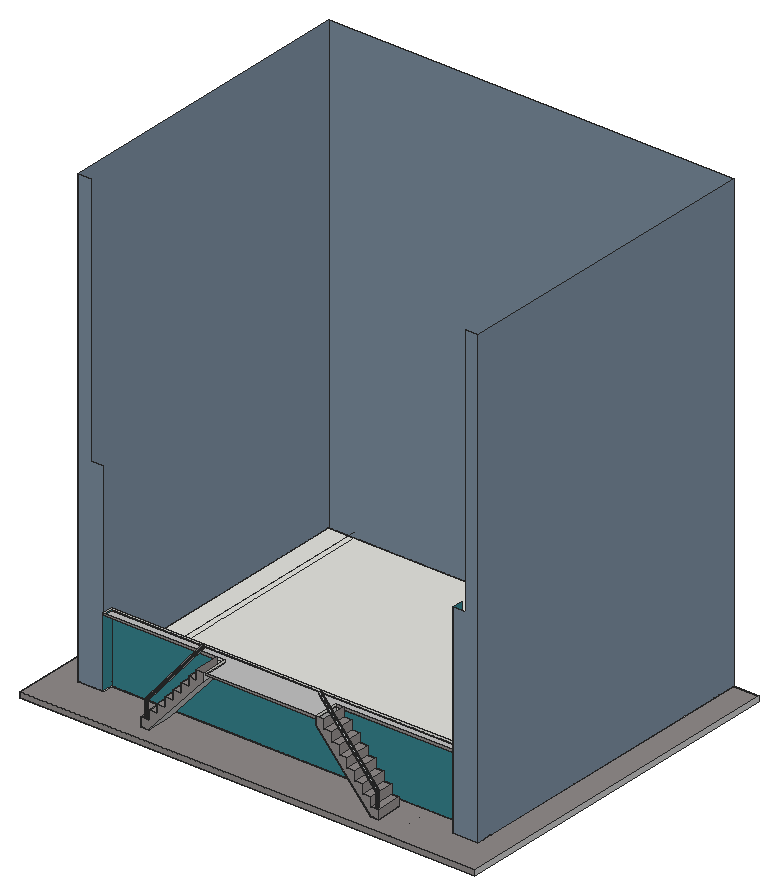
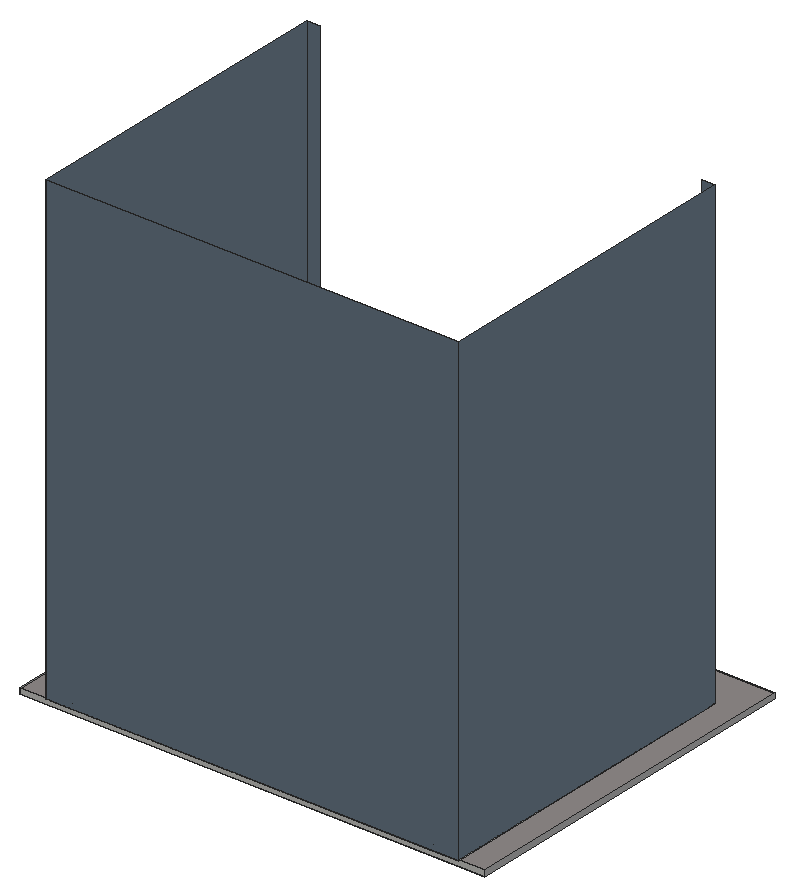
# SketchUp Ruby script. Lengths in inches.
U = 1.inch
M = Sketchup.active_model
def pt(a) = Geom::Point3d.new(a.map { |v| v * U })
def face(e, loops, mat)
  f = e.add_face(loops[0].map { |a| pt(a) })
  loops[1..].each { |l| e.add_face(l.map { |a| pt(a) }).erase! }
  f.material = f.back_material = mat if mat
  f
end
# faces: each face lists its corners as indices into pts; further lists are holes
def faces(e, pts, list, mat = nil) = list.each { |f| face(e, (f[0].is_a?(Array) ? f : [f]).map { |l| l.map { |i| pts[i] } }, mat) }
# xy, xz, yz: faces in a plane at the given z, y or x. An outline is a flat list of corners, or four numbers for a rectangle; further outlines are holes
def ring(l) = l.size == 4 ? [[l[0], l[1]], [l[2], l[1]], [l[2], l[3]], [l[0], l[3]]] : l.each_slice(2).to_a
def flat(e, list, mat, &to3) = list.each { |f| face(e, (f[0].is_a?(Array) ? f : [f]).map { |l| ring(l).map { |u, v| to3.(u, v) } }, mat) }
def xy(e, z, list, mat = nil) = flat(e, list, mat) { |x, y| [x, y, z] }
def xz(e, y, list, mat = nil) = flat(e, list, mat) { |x, z| [x, y, z] }
def yz(e, x, list, mat = nil) = flat(e, list, mat) { |y, z| [x, y, z] }
def lines(e, pts, list) = list.each { |a, b| e.add_line(pt(pts[a]), pt(pts[b])) }
# prism: a flat outline (further loops are holes) pulled along v
def prism(e, loops, v, mat = nil)
  f = face(e, loops, mat); d = Geom::Vector3d.new(v.map { |x| x * U })
  f.pushpull(f.normal.samedirection?(d) ? d.length : -d.length)
end
def box(e, o, s, mat = nil) = prism(e, [[o, [o[0] + s[0], o[1], o[2]], [o[0] + s[0], o[1] + s[1], o[2]], [o[0], o[1] + s[1], o[2]]]], [0, 0, s[2]], mat)
def at(x, y, z, deg = 0) = Geom::Transformation.translation(pt([x, y, z])) * Geom::Transformation.rotation(ORIGIN, Z_AXIS, deg.degrees)
def axes(o, x, y, z) = Geom::Transformation.new([*x, 0, *y, 0, *z, 0, *pt(o).to_a, 1])
def part(name) = M.definitions.add(name)
# library, detail: a bought-in or finely detailed component or shape, given as its bounding box
def library(name, o, s) = part(name).tap { |d| box(d.entities, o, s) }
def detail(e, o, s) = box(e.add_group.entities, o, s)
def put(e, d, t, mat = nil) = e.add_instance(d, t).tap { |i| i.material = mat if mat }
def group(e, t, mat = nil) = e.add_group.tap { |g| g.transformation = t; g.material = mat if mat }.entities
root = M.entities
M.materials.add("[0083_DarkTurquoise]").color = [52, 127, 137]
M.materials.add("[0110_LightSlateGray]").color = [119, 136, 153]
M.materials.add("[0131_Silver]").color = [192, 192, 192]
M.materials.add("[Steel Brushed Stainless]").color = [183, 187, 190]
M.materials.add("[Stone Marble]").color = [143, 138, 136]
xy(root,-12,[[0,0,1080,841.201]])
xy(root,0,[[60,97.201,120,121.201],[960,97.201,1020,121.201],[60,121.201,120,841.201],[120,121.201,960,841.201],[960,121.201,1020,841.201]])
xy(root,0.499,[[960,83.889,1020,97.201]])
xy(root,0.499,[[[0,0,1080,0,1080,841.201,1020,841.201,1020,83.889,960,83.889,960,121.201,120,121.201,120,97.201,60,97.201,60,841.201,0,841.201],[258.4,36.241,277.1,97.201],[802.9,37.201,821.6,98.161]]],"[Stone Marble]")
xy(root,0.5,[[258.4,36.241,277.1,97.201],[802.9,37.201,821.6,98.161]])
xy(root,21.4375,[[266.14,39.152,265.375,39.322,264.68,39.683,264.103,40.213,263.682,40.873,263.447,41.62,263.413,42.403,263.583,43.167,263.945,43.862,264.474,44.439,265.134,44.86,265.881,45.095,266.664,45.129,267.428,44.959,268.123,44.598,268.7,44.068,269.121,43.408,269.356,42.661,269.39,41.878,269.221,41.114,268.859,40.419,268.329,39.842,267.669,39.421,266.922,39.186]])
xy(root,21.4375,[[[258.4,36.241,277.1,97.201],[266.14,39.152,265.375,39.322,264.68,39.683,264.103,40.213,263.682,40.873,263.447,41.62,263.413,42.403,263.583,43.167,263.945,43.862,264.474,44.439,265.134,44.86,265.881,45.095,266.664,45.129,267.428,44.959,268.123,44.598,268.7,44.068,269.121,43.408,269.356,42.661,269.39,41.878,269.221,41.114,268.859,40.419,268.329,39.842,267.669,39.421,266.922,39.186]],[[802.9,37.201,821.6,98.161],[814.759,38.369,813.977,38.406,813.231,38.643,812.571,39.066,812.044,39.645,811.684,40.34,811.516,41.105,811.553,41.887,811.79,42.634,812.213,43.293,812.792,43.821,813.487,44.181,814.252,44.348,815.034,44.312,815.781,44.074,816.44,43.652,816.968,43.073,817.328,42.377,817.495,41.612,817.459,40.83,817.221,40.084,816.799,39.424,816.22,38.897,815.524,38.537]]],"[Stone Marble]")
xy(root,42.375,[[277.1,36.241,295.8,97.201],[784.2,37.201,802.9,98.161]],"[Stone Marble]")
xy(root,63.3125,[[295.8,36.241,314.5,97.201],[765.5,37.201,784.2,98.161]],"[Stone Marble]")
xy(root,84.25,[[314.5,36.241,333.2,97.201],[746.8,37.201,765.5,98.161]],"[Stone Marble]")
xy(root,105.1875,[[333.2,36.241,351.9,97.201],[728.1,37.201,746.8,98.161]],"[Stone Marble]")
xy(root,126.125,[[351.9,36.241,370.6,97.201],[709.4,37.201,728.1,98.161]],"[Stone Marble]")
xy(root,147.0625,[[370.6,36.241,389.3,97.201],[690.7,37.201,709.4,98.161]],"[Stone Marble]")
xy(root,162,[[408,37.201,408,97.201,120,97.201,120,121.201,960,121.201,960,97.201,672,97.201,672,37.201]],"[0131_Silver]")
xz(root,0,[[900,0.497,902.927,0.499,876,0.499],[875.998,0.499,875.998,0.5,876,0.499],[875.998,0.499,876,0.499,875.998,0.5],[876,0.499,875.998,0.5,876,0.5],[876,0.499,876,0.5,875.998,0.5],
  [876,0.499,876,0.5,875.998,0.5]])
xz(root,0,[[0,-12,1080,-12,1080,0.499,902.927,0.499,900,0.497,876,0.499,0,0.499]],"[Stone Marble]")
xz(root,36.241,[[258.4,0.499,277.1,0.5]])
xz(root,36.241,[[258.4,0.5,277.1,0.5,408,149.389,408,168,389.3,168,389.3,147.0625,370.6,147.0625,370.6,126.125,351.9,126.125,351.9,105.1875,333.2,105.1875,333.2,84.25,314.5,84.25,314.5,63.3125,295.8,63.3125,295.8,42.375,277.1,42.375,277.1,21.4375,258.4,21.4375]],"[Stone Marble]")
xz(root,37.201,[[802.9,0.499,821.6,0.5]])
xz(root,37.201,[[802.9,0.5,821.6,0.5,821.6,21.4375,802.9,21.4375,802.9,42.375,784.2,42.375,784.2,63.3125,765.5,63.3125,765.5,84.25,746.8,84.25,746.8,105.1875,728.1,105.1875,728.1,126.125,709.4,126.125,709.4,147.0625,690.7,147.0625,690.7,168,672,168,672,149.389],[408,162,672,168]],"[Stone Marble]")
xz(root,83.889,[[960,0.499,1020,0.499,1020,1080,990,1080,990,480,960,480]],"[0110_LightSlateGray]")
xz(root,97.201,[[60,0,120,0.499],[960,0,1020,0.499],[258.4,0.499,277.1,0.5],[258.4,0.5,258.4,21.4375,277.1,21.4375,277.1,42.375,295.8,42.375,295.8,63.3125,314.5,63.3125,314.5,84.25,333.2,84.25,333.2,105.1875,351.9,105.1875,351.9,126.125,370.6,126.125,370.6,147.0625,389.3,147.0625,389.3,162,408,162,408,149.389,277.1,0.5],[389.3,162,408,168]])
xz(root,97.201,[[60,0.499,120,0.499,120,480,90,480,90,1080,60,1080]],"[0110_LightSlateGray]")
xz(root,97.201,[[120,162,389.3,168],[672,162,960,168]],"[Stone Marble]")
xz(root,98.161,[[802.9,0.499,821.6,0.5],[802.9,0.5,672,149.389,672,162,690.7,162,690.7,147.0625,709.4,147.0625,709.4,126.125,728.1,126.125,728.1,105.1875,746.8,105.1875,746.8,84.25,765.5,84.25,765.5,63.3125,784.2,63.3125,784.2,42.375,802.9,42.375,802.9,21.4375,821.6,21.4375,821.6,0.5],[672,162,690.7,168]])
xz(root,121.201,[[120,0,960,0.499],[120,162,960,162,960,168,672,168,672,167.95,648,167.95,648,168,120,168]])
xz(root,121.201,[[120,0.499,960,162]],"[0083_DarkTurquoise]")
xz(root,841.201,[[0,-12,0,0.499,60,0.499,60,0,1020,0,1020,0.499,1080,0.499,1080,-12]])
xz(root,841.201,[[60,0,1020,1080]],"[0110_LightSlateGray]")
yz(root,0,[[0,-12,841.201,0.499]],"[0131_Silver]")
yz(root,60,[[97.201,0,121.201,0.499],[121.201,0,841.201,0.499]])
yz(root,60,[[97.201,0.499,841.201,1080]],"[0110_LightSlateGray]")
yz(root,120,[[97.201,0,121.201,0.499],[97.201,162,121.201,168]])
yz(root,120,[[97.201,0.499,121.201,162]],"[0083_DarkTurquoise]")
yz(root,258.4,[[36.241,0.499,97.201,0.5]])
yz(root,258.4,[[36.241,0.5,97.201,21.4375]],"[Stone Marble]")
yz(root,277.1,[[36.241,0.499,97.201,0.5]])
yz(root,277.1,[[36.241,21.4375,97.201,42.375]],"[Stone Marble]")
yz(root,295.8,[[36.241,42.375,97.201,63.3125]],"[Stone Marble]")
yz(root,314.5,[[36.241,63.3125,97.201,84.25]],"[Stone Marble]")
yz(root,333.2,[[36.241,84.25,97.201,105.1875]],"[Stone Marble]")
yz(root,351.9,[[36.241,105.1875,97.201,126.125]],"[Stone Marble]")
yz(root,370.6,[[36.241,126.125,97.201,147.0625]],"[Stone Marble]")
yz(root,389.3,[[36.241,147.0625,97.201,168]],"[Stone Marble]")
yz(root,408,[[37.201,162,97.201,168]])
yz(root,408,[[36.241,149.389,97.201,149.389,97.201,162,37.201,162,37.201,168,36.241,168]],"[0131_Silver]")
yz(root,672,[[37.201,162,97.201,168],[97.201,162,98.161,168]])
yz(root,672,[[37.201,149.389,98.161,162]],"[0131_Silver]")
yz(root,690.7,[[37.201,147.0625,98.161,168]],"[Stone Marble]")
yz(root,709.4,[[37.201,126.125,98.161,147.0625]],"[Stone Marble]")
yz(root,728.1,[[37.201,105.1875,98.161,126.125]],"[Stone Marble]")
yz(root,746.8,[[37.201,84.25,98.161,105.1875]],"[Stone Marble]")
yz(root,765.5,[[37.201,63.3125,98.161,84.25]],"[Stone Marble]")
yz(root,784.2,[[37.201,42.375,98.161,63.3125]],"[Stone Marble]")
yz(root,802.9,[[37.201,0.499,98.161,0.5]])
yz(root,802.9,[[37.201,21.4375,98.161,42.375]],"[Stone Marble]")
yz(root,821.6,[[37.201,0.499,98.161,0.5]])
yz(root,821.6,[[37.201,0.5,98.161,21.4375]],"[Stone Marble]")
yz(root,960,[[97.201,0,121.201,0.499],[97.201,162,121.201,168]])
yz(root,960,[[83.889,0.499,83.889,480,109.201,480,109.201,408,121.201,408,121.201,168,97.201,168,97.201,162,121.201,162,121.201,0.499]],"[0083_DarkTurquoise]")
yz(root,1020,[[97.201,0,121.201,0.499],[121.201,0,841.201,0.499]])
yz(root,1020,[[83.889,0.499,841.201,1080]],"[0110_LightSlateGray]")
yz(root,1080,[[0,-12,841.201,0.499]],"[0131_Silver]")
p = [[277.1,97.201,0.5],[408,97.201,149.389],[408,36.241,149.389],[277.1,36.241,0.5],[802.9,37.201,0.5],[672,37.201,149.389],
  [672,98.161,149.389],[802.9,98.161,0.5],[813.977,38.406,57.264],[813.231,38.643,56.982],[813.231,38.643,21.4375],[813.977,38.406,21.4375],
  [814.759,38.369,57.558],[814.759,38.369,21.4375],[815.524,38.537,57.844],[815.524,38.537,21.4375],[816.22,38.897,58.102],[816.22,38.897,21.4375],
  [812.571,39.066,56.731],[812.571,39.066,21.4375],[816.799,39.424,58.315],[816.799,39.424,21.4375],[812.044,39.645,56.528],[812.044,39.645,21.4375],
  [265.375,39.322,21.4375],[266.14,39.152,21.4375],[266.14,39.152,57.552],[265.375,39.322,57.828],[266.922,39.186,21.4375],[266.922,39.186,57.268],
  [267.669,39.421,21.4375],[267.669,39.421,56.996],[264.68,39.683,21.4375],[264.68,39.683,58.077],[268.329,39.842,21.4375],[268.329,39.842,56.754],
  [817.221,40.084,58.468],[817.221,40.084,21.4375],[811.684,40.34,56.387],[811.684,40.34,21.4375],[264.103,40.213,21.4375],[264.103,40.213,58.283],
  [268.859,40.419,21.4375],[268.859,40.419,56.558],[817.459,40.83,58.551],[817.459,40.83,21.4375],[263.682,40.873,21.4375],[263.682,40.873,58.431],
  [811.516,41.105,56.317],[811.516,41.105,21.4375],[269.221,41.114,21.4375],[269.221,41.114,56.422],[817.495,41.612,58.558],[817.495,41.612,21.4375],
  [263.447,41.62,21.4375],[263.447,41.62,58.512],[269.39,41.878,21.4375],[269.39,41.878,56.356],[811.553,41.887,56.324],[811.553,41.887,21.4375],
  [263.413,42.403,21.4375],[263.413,42.403,58.519],[817.328,42.377,58.488],[817.328,42.377,21.4375],[269.356,42.661,21.4375],[269.356,42.661,56.363],
  [811.79,42.634,56.407],[811.79,42.634,21.4375],[263.583,43.167,21.4375],[263.583,43.167,58.453],[816.968,43.073,58.347],[816.968,43.073,21.4375],
  [812.213,43.293,56.56],[812.213,43.293,21.4375],[269.121,43.408,21.4375],[269.121,43.408,56.444],[816.44,43.652,58.144],[816.44,43.652,21.4375],
  [263.945,43.862,21.4375],[263.945,43.862,58.317],[812.792,43.821,56.773],[812.792,43.821,21.4375],[268.7,44.068,21.4375],[268.7,44.068,56.592],
  [815.781,44.074,57.893],[815.781,44.074,21.4375],[813.487,44.181,57.031],[813.487,44.181,21.4375],[264.474,44.439,21.4375],[264.474,44.439,58.121],
  [268.123,44.598,21.4375],[268.123,44.598,56.798],[815.034,44.312,57.611],[815.034,44.312,21.4375],[814.252,44.348,57.317],[814.252,44.348,21.4375],
  [265.134,44.86,21.4375],[265.134,44.86,57.879],[267.428,44.959,21.4375],[267.428,44.959,57.047],[265.881,45.095,21.4375],[265.881,45.095,57.607],
  [266.664,45.129,21.4375],[266.664,45.129,57.323],[674.584,43.467,213.191],[674.511,44.23,213.014],[674.53,45.013,213.041],[674.64,45.762,213.269],
  [674.745,42.776,213.56],[400.066,43.467,213.191],[399.898,42.776,213.56],[400.143,44.23,213.014],[400.125,45.013,213.041],[674.834,46.427,213.683],
  [400.013,45.762,213.269],[399.815,46.427,213.683],[674.983,42.204,214.094],[399.652,42.204,214.094],[675.099,46.962,214.255],[399.543,46.962,214.255],
  [675.281,41.79,214.759],[399.344,41.79,214.759],[675.416,47.33,214.946],[399.217,47.33,214.946],[675.619,41.562,215.508],[398.995,41.562,215.508],
  [675.764,47.507,215.709],[398.859,47.507,215.709],[675.974,41.535,216.291],[398.629,41.535,216.291],[676.119,47.481,216.492],[398.493,47.481,216.492],
  [676.322,41.712,217.054],[398.271,41.712,217.054],[676.457,47.252,217.241],[398.144,47.252,217.241],[676.639,42.081,217.745],[397.945,42.081,217.745],
  [676.755,46.838,217.906],[397.836,46.838,217.906],[676.903,42.615,218.317],[397.673,42.615,218.317],[676.993,46.266,218.44],[397.59,46.266,218.44],
  [677.098,43.28,218.731],[397.475,43.28,218.731],[677.154,45.575,218.809],[397.422,45.575,218.809],[397.363,44.029,218.959],[677.208,44.029,218.959],
  [397.345,44.812,218.986],[677.227,44.812,218.986],[672,97.201,162],[672,37.201,162],[672.031,37.201,162.039],[672.031,97.201,162.039],
  [120,841.201,12],[120,121.201,12],[960,121.201,12],[960,841.201,12],[876,60.601,0.499],[876.031,60.601,0.538],
  [875.998,90.3,0.5],[876.029,90.3,0.539],[814.506,41.359,21.4375],[814.506,41.359,57.4375],[266.402,42.14,21.4375],[266.402,42.14,57.4375],
  [398.744,44.521,216],[675.869,44.521,216],[960,0,0.55],[902.927,0,0.5]]
faces(root,p,[[0,1,2,3],[4,5,6,7]],"[0131_Silver]")
faces(root,p,[[8,9,10,11],[12,8,11,13],[14,12,13,15],[16,14,15,17],[9,18,19,10],[20,16,17,21],[18,22,23,19],[24,25,26,27],
  [25,28,29,26],[28,30,31,29],[32,24,27,33],[30,34,35,31],[36,20,21,37],[22,38,39,23],[40,32,33,41],[34,42,43,35],
  [44,36,37,45],[46,40,41,47],[38,48,49,39],[42,50,51,43],[52,44,45,53],[54,46,47,55],[50,56,57,51],[48,58,59,49],
  [60,54,55,61],[62,52,53,63],[56,64,65,57],[58,66,67,59],[68,60,61,69],[70,62,63,71],[66,72,73,67],[64,74,75,65],
  [76,70,71,77],[78,68,69,79],[72,80,81,73],[74,82,83,75],[84,76,77,85],[80,86,87,81],[88,78,79,89],[82,90,91,83],
  [92,84,85,93],[86,94,95,87],[94,92,93,95],[96,88,89,97],[90,98,99,91],[100,96,97,101],[98,102,103,99],[102,100,101,103],
  [104,105,48,38],[105,106,58,48],[106,107,66,58],[108,104,38,22],[43,51,109,110],[51,57,111,109],[57,65,112,111],[107,113,72,66],
  [65,75,114,112],[75,83,115,114],[116,108,22,18],[35,43,110,117],[113,118,80,72],[83,91,119,115],[120,116,18,9],[31,35,117,121],
  [118,122,86,80],[91,99,123,119],[124,120,9,8],[29,31,121,125],[122,126,94,86],[99,103,127,123],[128,124,8,12],[26,29,125,129],
  [126,130,92,94],[103,101,131,127],[132,128,12,14],[27,26,129,133],[130,134,84,92],[101,97,135,131],[136,132,14,16],[33,27,133,137],
  [134,138,76,84],[97,89,139,135],[140,136,16,20],[41,33,137,141],[138,142,70,76],[89,79,143,139],[144,140,20,36],[47,41,141,145],
  [142,146,62,70],[79,69,147,143],[55,47,145,148],[149,144,36,44],[61,55,148,150],[146,151,52,62],[69,61,150,147],[151,149,44,52]],"[Steel Brushed Stainless]")
faces(root,p,[[152,153,154,155]])
lines(root,p,[[156,157],[158,159],[160,161],[162,163],[164,165],[166,167],[167,168],[165,169],[170,171]])
